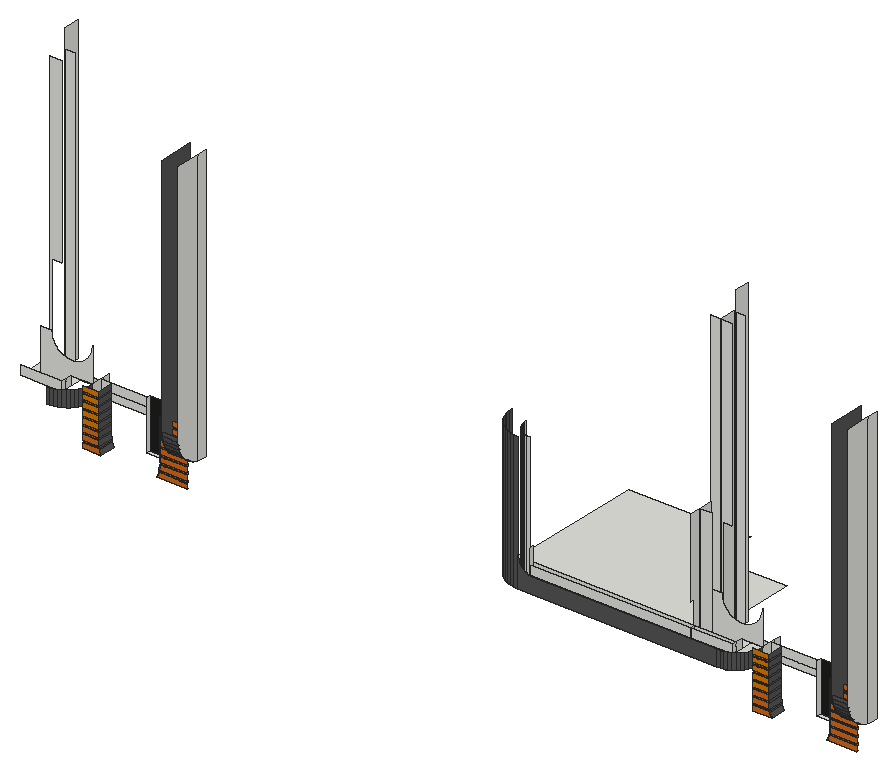
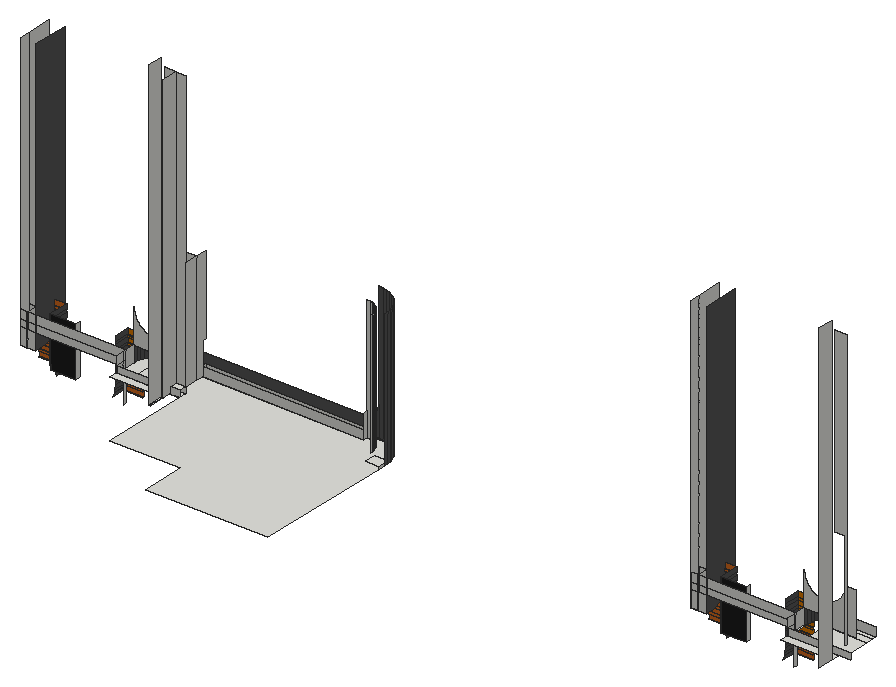
# SketchUp Ruby script. Lengths in inches.
U = 1.inch
M = Sketchup.active_model
def pt(a) = Geom::Point3d.new(a.map { |v| v * U })
def face(e, loops, mat)
  f = e.add_face(loops[0].map { |a| pt(a) })
  loops[1..].each { |l| e.add_face(l.map { |a| pt(a) }).erase! }
  f.material = f.back_material = mat if mat
  f
end
# faces: each face lists its corners as indices into pts; further lists are holes
def faces(e, pts, list, mat = nil) = list.each { |f| face(e, (f[0].is_a?(Array) ? f : [f]).map { |l| l.map { |i| pts[i] } }, mat) }
# xy, xz, yz: faces in a plane at the given z, y or x. An outline is a flat list of corners, or four numbers for a rectangle; further outlines are holes
def ring(l) = l.size == 4 ? [[l[0], l[1]], [l[2], l[1]], [l[2], l[3]], [l[0], l[3]]] : l.each_slice(2).to_a
def flat(e, list, mat, &to3) = list.each { |f| face(e, (f[0].is_a?(Array) ? f : [f]).map { |l| ring(l).map { |u, v| to3.(u, v) } }, mat) }
def xy(e, z, list, mat = nil) = flat(e, list, mat) { |x, y| [x, y, z] }
def xz(e, y, list, mat = nil) = flat(e, list, mat) { |x, z| [x, y, z] }
def yz(e, x, list, mat = nil) = flat(e, list, mat) { |y, z| [x, y, z] }
def lines(e, pts, list) = list.each { |a, b| e.add_line(pt(pts[a]), pt(pts[b])) }
# prism: a flat outline (further loops are holes) pulled along v
def prism(e, loops, v, mat = nil)
  f = face(e, loops, mat); d = Geom::Vector3d.new(v.map { |x| x * U })
  f.pushpull(f.normal.samedirection?(d) ? d.length : -d.length)
end
def box(e, o, s, mat = nil) = prism(e, [[o, [o[0] + s[0], o[1], o[2]], [o[0] + s[0], o[1] + s[1], o[2]], [o[0], o[1] + s[1], o[2]]]], [0, 0, s[2]], mat)
def at(x, y, z, deg = 0) = Geom::Transformation.translation(pt([x, y, z])) * Geom::Transformation.rotation(ORIGIN, Z_AXIS, deg.degrees)
def axes(o, x, y, z) = Geom::Transformation.new([*x, 0, *y, 0, *z, 0, *pt(o).to_a, 1])
def part(name) = M.definitions.add(name)
# library, detail: a bought-in or finely detailed component or shape, given as its bounding box
def library(name, o, s) = part(name).tap { |d| box(d.entities, o, s) }
def detail(e, o, s) = box(e.add_group.entities, o, s)
def put(e, d, t, mat = nil) = e.add_instance(d, t).tap { |i| i.material = mat if mat }
def group(e, t, mat = nil) = e.add_group.tap { |g| g.transformation = t; g.material = mat if mat }.entities
root = M.entities
M.materials.add("[0039_DarkOrange]").color = [219, 120, 0]
M.materials.add("[0041_Chocolate]").color = [210, 105, 30]
M.materials.add("[Color M06]").color = [84, 84, 84]
M.materials.add("[Color M08]").color = [30, 30, 30]
xy(root,90.875,[[1547.71,280.47,1565.89,281.47],[1619.87,280.47,1649.14,281.47],[2198.21,280.47,2216.39,281.47],[2270.37,280.47,2299.64,281.47]],"[0041_Chocolate]")
xy(root,95.83,[[1547.71,280.47,1564.03,281.47],[1621.74,280.47,1649.14,281.47],[2198.21,280.47,2214.53,281.47],[2272.24,280.47,2299.64,281.47]],"[0041_Chocolate]")
xy(root,97.27,[[1597.48,295.65,1621.93,300.34],[2247.98,295.65,2272.43,300.34]])
xy(root,97.9375,[[1547.71,280.47,1563.75,281.47],[1622.02,280.47,1649.14,281.47],[2198.21,280.47,2214.25,281.47],[2272.52,280.47,2299.64,281.47]],"[0041_Chocolate]")
xy(root,102.89,[[1547.71,280.47,1563.1,281.47],[1622.67,280.47,1649.14,281.47],[2198.21,280.47,2213.6,281.47],[2273.17,280.47,2299.64,281.47]],"[0041_Chocolate]")
xy(root,105,[[1547.71,280.47,1563.1,281.47],[1622.67,280.47,1649.14,281.47],[2198.21,280.47,2213.6,281.47],[2273.17,280.47,2299.64,281.47]],"[0041_Chocolate]")
xy(root,109.9375,[[1634.68,299.11,1650.02,302.46],[2285.18,299.11,2300.52,302.46]])
xy(root,109.95,[[1547.71,280.47,1563.1,281.47],[1622.67,280.47,1649.14,281.47],[2198.21,280.47,2213.6,281.47],[2273.17,280.47,2299.64,281.47]],"[0041_Chocolate]")
xy(root,112.0625,[[1547.71,280.47,1563.1,281.47],[2198.21,280.47,2213.6,281.47]],"[0039_DarkOrange]")
xy(root,112.0625,[[1622.67,280.47,1649.14,281.47],[2273.17,280.47,2299.64,281.47]],"[0041_Chocolate]")
xy(root,117.02,[[1547.71,280.47,1563.1,281.47],[2198.21,280.47,2213.6,281.47]],"[0039_DarkOrange]")
xy(root,117.02,[[1622.67,280.47,1649.14,281.47],[2273.17,280.47,2299.64,281.47]],"[0041_Chocolate]")
xy(root,119.125,[[1547.71,280.47,1563.1,281.47],[2198.21,280.47,2213.6,281.47]],"[0039_DarkOrange]")
xy(root,119.125,[[1622.67,280.47,1649.14,281.47],[2273.17,280.47,2299.64,281.47]],"[0041_Chocolate]")
xy(root,124.08,[[1547.71,280.47,1563.1,281.47],[2198.21,280.47,2213.6,281.47]],"[0039_DarkOrange]")
xy(root,124.08,[[1622.67,280.47,1649.14,281.47],[2273.17,280.47,2299.64,281.47]],"[0041_Chocolate]")
xy(root,126.125,[[1980.54,267.75,1976.54,268.01,1972.61,268.79,1970.16,269.625,2182.95,269.625,2179.9,268.59,2176.73,267.96,2173.51,267.75],[1970.16,269.625,1968.8125,270.08,1965.22,271.85,1961.88,274.08,1958.87,276.72,1957.13,278.71,1956.23,279.74,1954,283.07,1952.23,286.66,1950.94,290.46,1950.16,294.39,1949.9,298.39,1949.9,439.98,2068.38,439.98,2068.38,397.86,2137,397.86,2137,305.58,2146.71,305.58,2146.71,312.8125,2198.21,312.8125,2198.21,305.58,2197.71,305.58,2197.71,292.45,2198.21,292.45,2198,289.23,2197.37,286.06,2196.33,283,2194.9,280.1,2193.11,277.41,2190.98,274.98,2188.55,272.85,2185.86,271.06,2182.96,269.63,2182.95,269.625],[1547.21,292.45,1547.71,302.46],[2197.71,292.45,2198.21,302.46],[1547.21,302.46,1547.71,305.58],
  [2197.71,302.46,2198.21,305.58],[2137,305.58,2146.71,312.8125],[1498.09,312.8125,1507.74,321.34],[1507.74,312.8125,1547.71,321.34],[2146.71,312.8125,2147.02,321.34],
  [2147.02,312.8125,2148.59,321.34],[2148.59,312.8125,2158.24,321.34],[2158.24,312.8125,2198.21,321.34],[2146.71,321.34,2147.02,336.27],[2147.02,321.34,2148.59,336.27]])
xy(root,126.1875,[[1547.71,280.47,1563.1,281.47],[2198.21,280.47,2213.6,281.47]],"[0039_DarkOrange]")
xy(root,126.1875,[[1622.67,280.47,1649.14,281.47],[2273.17,280.47,2299.64,281.47]],"[0041_Chocolate]")
xy(root,128.75,[[1949.9,294.33,1962.9,305.58]])
xy(root,131.14,[[1547.71,280.47,1563.1,281.47],[2198.21,280.47,2213.6,281.47]],"[0039_DarkOrange]")
xy(root,131.14,[[1622.67,280.47,1649.14,281.47],[2273.17,280.47,2299.64,281.47]],"[0041_Chocolate]")
xy(root,132.47,[[1486.5,281.47,1527.09,285.84],[1980.54,281.47,2137,285.84],[2137,281.47,2177.59,285.84],[1486.5,285.84,1527.09,292.45],[2137,285.84,2177.59,292.45],
  [1486.5,292.45,1527.09,312.8125],[2137,292.45,2177.59,312.8125]])
xy(root,133.25,[[1547.71,280.47,1563.1,281.47],[2198.21,280.47,2213.6,281.47]],"[0039_DarkOrange]")
xy(root,133.25,[[1622.67,280.47,1649.14,281.47],[2273.17,280.47,2299.64,281.47]],"[0041_Chocolate]")
xy(root,138.2,[[1547.71,280.47,1563.1,281.47],[2198.21,280.47,2213.6,281.47]],"[0039_DarkOrange]")
xy(root,138.2,[[1622.67,280.47,1649.14,281.47],[2273.17,280.47,2299.64,281.47]],"[0041_Chocolate]")
xy(root,140.3125,[[1547.71,280.47,1563.1,281.47],[2198.21,280.47,2213.6,281.47]],"[0039_DarkOrange]")
xy(root,140.3125,[[1622.67,280.47,1649.14,281.47],[2273.17,280.47,2299.64,281.47]],"[0041_Chocolate]")
xz(root,267.75,[[1980.54,126.125,2173.51,126.125,2173.51,141.26,1993.98,141.26,1992.2,141.46,1990.46,141.89,1988.79,142.53,1987.21,143.38,1985.75,144.42,1984.43,145.64,1983.28,147.01,1982.32,148.52,1981.55,150.14,1980.99,151.84,1980.65,153.6,1980.54,155.39]],"[Color M06]")
xz(root,280.47,[[1547.71,112.0625,1563.1,117.02],[2198.21,112.0625,2213.6,117.02],[1547.71,119.125,1563.1,124.08],[2198.21,119.125,2213.6,124.08],[1547.71,126.1875,1563.1,131.14],
  [2198.21,126.1875,2213.6,131.14],[1547.71,133.25,1563.1,138.2],[2198.21,133.25,2213.6,138.2],[1547.71,140.3125,1563.1,145.27],[2198.21,140.3125,2213.6,145.27]],"[0039_DarkOrange]")
xz(root,280.47,[[1547.71,90.875,1565.89,90.875,1564.11,95.18,1564.03,95.83,1547.71,95.83],[1619.87,90.875,1649.14,90.875,1649.14,95.83,1621.74,95.83,1621.66,95.18],[2198.21,90.875,2216.39,90.875,2214.61,95.18,2214.53,95.83,2198.21,95.83],[2270.37,90.875,2299.64,90.875,2299.64,95.83,2272.24,95.83,2272.16,95.18],[1547.71,97.9375,1563.75,97.9375,1563.1,102.89,1547.71,102.89],
  [1622.02,97.9375,1649.14,97.9375,1649.14,102.89,1622.67,102.89],[2198.21,97.9375,2214.25,97.9375,2213.6,102.89,2198.21,102.89],[2272.52,97.9375,2299.64,97.9375,2299.64,102.89,2273.17,102.89],[1547.71,105,1563.1,109.95],[1622.67,105,1649.14,109.95],
  [2198.21,105,2213.6,109.95],[2273.17,105,2299.64,109.95],[1622.67,112.0625,1649.14,117.02],[2273.17,112.0625,2299.64,117.02],[1622.67,119.125,1649.14,124.08],
  [2273.17,119.125,2299.64,124.08],[1622.67,126.1875,1649.14,131.14],[2273.17,126.1875,2299.64,131.14],[1622.67,133.25,1649.14,138.2],[2273.17,133.25,2299.64,138.2],
  [1622.67,140.3125,1649.14,145.27],[2273.17,140.3125,2299.64,145.27]],"[0041_Chocolate]")
xz(root,281.47,[[1486.5,132.47,1527.09,141.26],[1980.54,132.47,2137,141.26],[2137,132.47,2177.59,141.26]])
xz(root,281.47,[[1547.71,117.02,1563.1,119.125],[2198.21,117.02,2213.6,119.125],[1547.71,124.08,1563.1,126.1875],[2198.21,124.08,2213.6,126.1875],[1547.71,131.14,1563.1,133.25],
  [2198.21,131.14,2213.6,133.25],[1547.71,138.2,1563.1,140.3125],[2198.21,138.2,2213.6,140.3125]],"[0039_DarkOrange]")
xz(root,281.47,[[1547.71,95.83,1564.03,95.83,1563.75,97.9375,1547.71,97.9375],[1621.74,95.83,1649.14,95.83,1649.14,97.9375,1622.02,97.9375],[2198.21,95.83,2214.53,95.83,2214.25,97.9375,2198.21,97.9375],[2272.24,95.83,2299.64,95.83,2299.64,97.9375,2272.52,97.9375],[1547.71,102.89,1563.1,105],
  [1622.67,102.89,1649.14,105],[2198.21,102.89,2213.6,105],[2273.17,102.89,2299.64,105],[1547.71,109.95,1563.1,112.0625],[1622.67,109.95,1649.14,112.0625],
  [2198.21,109.95,2213.6,112.0625],[2273.17,109.95,2299.64,112.0625],[1622.67,117.02,1649.14,119.125],[2273.17,117.02,2299.64,119.125],[1622.67,124.08,1649.14,126.1875],
  [2273.17,124.08,2299.64,126.1875],[1622.67,131.14,1649.14,133.25],[2273.17,131.14,2299.64,133.25],[1622.67,138.2,1649.14,140.3125],[2273.17,138.2,2299.64,140.3125]],"[0041_Chocolate]")
xz(root,285.84,[[1980.54,132.47,2177.59,141.26]])
xz(root,292.45,[[1642.35,126.125,1643.23,141.26],[1643.23,126.125,1649.14,141.26],[2292.85,126.125,2293.73,141.26],[2293.73,126.125,2299.64,141.26],[1498.09,132.47,1527.09,132.47,1527.09,141.26,1547.71,141.26,1547.71,174.51,1547.68,173.46,1547.6,172.42,1547.46,171.38,1547.27,170.36,1547.03,169.34,1546.73,168.33,1546.38,167.35,1545.98,166.38,1545.53,165.4375,1545.03,164.52,1544.49,163.625,1543.89,162.76,1543.26,161.93,1542.58,161.14,1541.86,160.38,1541.1,159.66,1540.3,158.98,1539.47,158.34,1538.61,157.75,1537.72,157.2,1536.8,156.7,1535.86,156.25,1534.89,155.85,1533.9,155.5,1532.9,155.21,1531.88,154.96,1530.85,154.77,1529.82,154.64,1528.77,154.55,1527.73,154.53,1526.68,154.55,1525.64,154.64,1524.6,154.77,1523.57,154.96,1522.55,155.21,1521.55,155.5,1520.57,155.85,1519.6,156.25,1518.65,156.7,1517.73,157.2,1516.84,157.75,1515.98,158.34,1515.15,158.98,1514.35,159.66,1513.6,160.38,1512.875,161.14,1512.2,161.93,1511.56,162.76,1510.97,163.625,1510.42,164.52,1509.92,165.4375,1509.47,166.38,1509.07,167.35,1508.72,168.33,1508.42,169.34,1508.18,170.36,1507.99,171.38,1507.85,172.42,1507.77,173.46,1507.74,174.51,1498.09,174.51],
  [2137,132.47,2148.59,240.16],[2148.59,132.47,2177.59,132.47,2177.59,141.26,2198.21,141.26,2198.21,174.51,2198.18,173.46,2198.1,172.42,2197.96,171.38,2197.77,170.36,2197.53,169.34,2197.23,168.33,2196.88,167.35,2196.48,166.38,2196.03,165.4375,2195.53,164.52,2194.99,163.625,2194.39,162.76,2193.76,161.93,2193.08,161.14,2192.36,160.38,2191.6,159.66,2190.8,158.98,2189.97,158.34,2189.11,157.75,2188.22,157.2,2187.3,156.7,2186.36,156.25,2185.39,155.85,2184.4,155.5,2183.4,155.21,2182.38,154.96,2181.35,154.77,2180.32,154.64,2179.27,154.55,2178.23,154.53,2177.18,154.55,2176.14,154.64,2175.1,154.77,2174.07,154.96,2173.05,155.21,2172.05,155.5,2171.07,155.85,2170.1,156.25,2169.15,156.7,2168.23,157.2,2167.34,157.75,2166.48,158.34,2165.65,158.98,2164.85,159.66,2164.1,160.38,2163.375,161.14,2162.7,161.93,2162.06,162.76,2161.47,163.625,2160.92,164.52,2160.42,165.4375,2159.97,166.38,2159.57,167.35,2159.22,168.33,2158.92,169.34,2158.68,170.36,2158.49,171.38,2158.35,172.42,2158.27,173.46,2158.24,174.51,2148.59,174.51]])
xz(root,295.65,[[1621.93,97.27,1622.67,97.27,1622.67,102.89,1622.02,97.9375],[2272.43,97.27,2273.17,97.27,2273.17,102.89,2272.52,97.9375]])
xz(root,300.34,[[1597.48,97.27,1621.93,97.27,1622.02,97.9375,1622.67,102.89,1622.67,145.27,1597.48,145.27],[2247.98,97.27,2272.43,97.27,2272.52,97.9375,2273.17,102.89,2273.17,145.27,2247.98,145.27]],"[Color M08]")
xz(root,302.46,[[1547.21,95.62,1547.71,126.125],[2197.71,95.62,2198.21,126.125],[1634.68,109.9375,1642.35,126.125],[1642.35,109.9375,1643.23,126.125],[1643.23,109.9375,1650.02,126.125],
  [2285.18,109.9375,2292.85,126.125],[2292.85,109.9375,2293.73,126.125],[2293.73,109.9375,2300.52,126.125],[1547.71,126.125,1634.68,132.47],[1634.68,126.125,1642.35,132.47],
  [1642.35,126.125,1643.23,132.47],[1643.23,126.125,1650.02,132.47],[2198.21,126.125,2285.18,132.47],[2285.18,126.125,2292.85,132.47],[2292.85,126.125,2293.73,132.47],
  [2293.73,126.125,2300.52,132.47],[1547.71,132.47,1634.68,141.26],[1634.68,132.47,1642.35,141.26],[1642.35,132.47,1643.23,141.26],[1643.23,132.47,1650.02,141.26],
  [2198.21,132.47,2285.18,141.26],[2285.18,132.47,2292.85,141.26],[2292.85,132.47,2293.73,141.26],[2293.73,132.47,2300.52,141.26]])
xz(root,305.58,[[1496.21,126.125,1498.09,126.125,1498.09,226.8,1507.74,226.8,1507.74,402.64,1496.21,402.64],[2137,126.125,2146.71,402.64],[2146.71,126.125,2148.59,126.125,2148.59,226.8,2158.24,226.8,2158.24,402.64,2146.71,402.64]])
xz(root,312.8125,[[1486.5,126.125,1547.71,132.47],[2137,126.125,2198.21,132.47]])
xz(root,321.34,[[1498.09,126.125,1507.74,402.64],[2146.71,126.125,2148.59,402.64],[2148.59,126.125,2158.24,402.64]])
yz(root,1498.09,[[321.34,126.125,336.27,421.25]])
yz(root,1527.09,[[281.47,132.47,285.84,141.26],[285.84,132.47,292.45,141.26]])
yz(root,1547.21,[[302.46,95.62,305.58,126.125]])
yz(root,1547.71,[[292.45,126.125,302.46,141.26],[302.46,126.125,305.58,132.47],[305.58,126.125,312.8125,132.47],[302.46,132.47,305.58,141.26],[305.58,132.47,312.8125,141.26]])
yz(root,1563.1,[[281.47,102.89,295.65,105],[280.47,105,295.65,109.95],[281.47,109.95,295.65,112.0625],[280.47,112.0625,295.65,117.02],[281.47,117.02,295.65,119.125],
  [280.47,119.125,295.65,124.08],[281.47,124.08,295.65,126.1875],[280.47,126.1875,295.65,131.14],[281.47,131.14,295.65,133.25],[280.47,133.25,295.65,138.2],
  [281.47,138.2,295.65,140.3125],[280.47,140.3125,295.65,145.27]],"[Color M06]")
yz(root,1597.48,[[295.65,97.27,300.34,145.27]])
yz(root,1622.67,[[281.47,102.89,300.34,105],[280.47,105,300.34,109.95],[281.47,109.95,300.34,112.0625],[280.47,112.0625,300.34,117.02],[281.47,117.02,300.34,119.125],
  [280.47,119.125,300.34,124.08],[281.47,124.08,300.34,126.1875],[280.47,126.1875,300.34,131.14],[281.47,131.14,300.34,133.25],[280.47,133.25,300.34,138.2],
  [281.47,138.2,300.34,140.3125],[280.47,140.3125,300.34,145.27]],"[Color M06]")
yz(root,1634.68,[[299.11,109.9375,295.02,110.21,290.99,111.01,287.11,112.32,283.43,114.14,280.02,116.42,276.93,119.12,274.23,122.21,271.95,125.62,270.14,129.3,268.82,133.18,268.02,137.2,267.75,141.3,267.75,376.875,302.46,376.875,302.46,109.9375]],"[Color M06]")
yz(root,1642.35,[[292.45,126.125,302.46,141.26]])
yz(root,1650.02,[[299.11,109.9375,302.46,109.9375,302.46,376.875,292.45,376.875,292.45,110.72,295.02,110.21],[299.11,109.9375,302.46,109.9375,302.46,376.875,292.45,376.875,292.45,110.72,295.02,110.21],[292.45,110.72,292.45,376.875,267.75,376.875,267.75,141.3,268.02,137.2,268.82,133.18,270.14,129.3,271.95,125.62,274.23,122.21,276.93,119.12,280.02,116.42,283.43,114.14,287.11,112.32,290.99,111.01]])
yz(root,1949.9,[[298.39,126.125,305.58,128.75]])
yz(root,1980.54,[[281.47,132.47,285.84,155.39]])
yz(root,2137,[[281.47,132.47,281.47,141.26,285.84,141.26,285.84,163.7,281.47,163.7,281.47,240.16,292.45,240.16,292.45,132.47],[292.45,132.47,305.58,240.16]])
yz(root,2146.71,[[305.58,126.125,321.34,402.64]])
yz(root,2148.59,[[321.34,126.125,336.27,421.25]])
yz(root,2177.59,[[281.47,132.47,285.84,141.26],[285.84,132.47,292.45,141.26]])
yz(root,2197.71,[[302.46,95.62,305.58,126.125]])
yz(root,2198.21,[[292.45,126.125,302.46,141.26],[302.46,126.125,305.58,132.47],[305.58,126.125,312.8125,132.47],[302.46,132.47,305.58,141.26],[305.58,132.47,312.8125,141.26]])
yz(root,2213.6,[[281.47,102.89,295.65,105],[280.47,105,295.65,109.95],[281.47,109.95,295.65,112.0625],[280.47,112.0625,295.65,117.02],[281.47,117.02,295.65,119.125],
  [280.47,119.125,295.65,124.08],[281.47,124.08,295.65,126.1875],[280.47,126.1875,295.65,131.14],[281.47,131.14,295.65,133.25],[280.47,133.25,295.65,138.2],
  [281.47,138.2,295.65,140.3125],[280.47,140.3125,295.65,145.27]],"[Color M06]")
yz(root,2247.98,[[295.65,97.27,300.34,145.27]])
yz(root,2273.17,[[281.47,102.89,300.34,105],[280.47,105,300.34,109.95],[281.47,109.95,300.34,112.0625],[280.47,112.0625,300.34,117.02],[281.47,117.02,300.34,119.125],
  [280.47,119.125,300.34,124.08],[281.47,124.08,300.34,126.1875],[280.47,126.1875,300.34,131.14],[281.47,131.14,300.34,133.25],[280.47,133.25,300.34,138.2],
  [281.47,138.2,300.34,140.3125],[280.47,140.3125,300.34,145.27]],"[Color M06]")
yz(root,2285.18,[[299.11,109.9375,295.02,110.21,290.99,111.01,287.11,112.32,283.43,114.14,280.02,116.42,276.93,119.12,274.23,122.21,271.95,125.62,270.14,129.3,268.82,133.18,268.02,137.2,267.75,141.3,267.75,376.875,302.46,376.875,302.46,109.9375]],"[Color M06]")
yz(root,2292.85,[[292.45,126.125,302.46,141.26]])
yz(root,2300.52,[[299.11,109.9375,302.46,109.9375,302.46,376.875,292.45,376.875,292.45,110.72,295.02,110.21],[292.45,110.72,292.45,376.875,267.75,376.875,267.75,141.3,268.02,137.2,268.82,133.18,270.14,129.3,271.95,125.62,274.23,122.21,276.93,119.12,280.02,116.42,283.43,114.14,287.11,112.32,290.99,111.01]])
p = [[1564.11,295.65,95.18],[1564.11,280.47,95.18],[1565.89,280.47,90.875],[1565.89,281.47,90.875],[1565.89,295.65,90.875],[1619.87,295.65,90.875],
  [1619.87,281.47,90.875],[1619.87,280.47,90.875],[1621.66,280.47,95.18],[1621.66,295.65,95.18],[2214.61,295.65,95.18],[2214.61,280.47,95.18],
  [2216.39,280.47,90.875],[2216.39,281.47,90.875],[2216.39,295.65,90.875],[2270.37,295.65,90.875],[2270.37,281.47,90.875],[2270.37,280.47,90.875],
  [2272.16,280.47,95.18],[2272.16,295.65,95.18],[1564.03,295.65,95.83],[1564.03,281.47,95.83],[1564.03,280.47,95.83],[1621.74,280.47,95.83],
  [1621.74,281.47,95.83],[1621.74,295.65,95.83],[2214.53,295.65,95.83],[2214.53,281.47,95.83],[2214.53,280.47,95.83],[2272.24,280.47,95.83],
  [2272.24,281.47,95.83],[2272.24,295.65,95.83],[1563.75,281.47,97.9375],[1563.75,295.65,97.9375],[1622.02,281.47,97.9375],[1622.02,295.65,97.9375],
  [1621.93,295.65,97.27],[2214.25,281.47,97.9375],[2214.25,295.65,97.9375],[2272.52,281.47,97.9375],[2272.52,295.65,97.9375],[2272.43,295.65,97.27],
  [1622.02,300.34,97.9375],[1621.93,300.34,97.27],[2272.52,300.34,97.9375],[2272.43,300.34,97.27],[1563.1,295.65,102.89],[1563.1,281.47,102.89],
  [1563.1,280.47,102.89],[1563.75,280.47,97.9375],[1622.02,280.47,97.9375],[1622.67,280.47,102.89],[1622.67,281.47,102.89],[1622.67,295.65,102.89],
  [2213.6,295.65,102.89],[2213.6,281.47,102.89],[2213.6,280.47,102.89],[2214.25,280.47,97.9375],[2272.52,280.47,97.9375],[2273.17,280.47,102.89],
  [2273.17,281.47,102.89],[2273.17,295.65,102.89],[1622.67,300.34,102.89],[2273.17,300.34,102.89],[1650.02,299.11,109.9375],[1650.02,295.02,110.21],
  [1634.68,295.02,110.21],[1634.68,299.11,109.9375],[2300.52,299.11,109.9375],[2300.52,295.02,110.21],[2285.18,295.02,110.21],[2285.18,299.11,109.9375],
  [1650.02,292.45,110.72],[1650.02,290.99,111.01],[1634.68,290.99,111.01],[2300.52,292.45,110.72],[2300.52,290.99,111.01],[2285.18,290.99,111.01],
  [1650.02,287.11,112.32],[1634.68,287.11,112.32],[2300.52,287.11,112.32],[2285.18,287.11,112.32],[1650.02,283.43,114.14],[1634.68,283.43,114.14],
  [2300.52,283.43,114.14],[2285.18,283.43,114.14],[1650.02,280.02,116.42],[1634.68,280.02,116.42],[2300.52,280.02,116.42],[2285.18,280.02,116.42],
  [1650.02,276.93,119.12],[1634.68,276.93,119.12],[2300.52,276.93,119.12],[2285.18,276.93,119.12],[1650.02,274.23,122.21],[1634.68,274.23,122.21],
  [2300.52,274.23,122.21],[2285.18,274.23,122.21],[1650.02,271.95,125.62],[1634.68,271.95,125.62],[2300.52,271.95,125.62],[2285.18,271.95,125.62],
  [1650.02,270.14,129.3],[1634.68,270.14,129.3],[2300.52,270.14,129.3],[2285.18,270.14,129.3],[1526.23,267.96,141.26],[1523.01,267.75,141.26],
  [1523.01,267.75,126.125],[1526.23,267.96,126.125],[1980.54,267.75,258.13],[1976.54,268.01,258.13],[1976.54,268.01,126.125],[1980.54,267.75,126.125],
  [1980.54,267.75,155.39],[1980.54,267.75,164.97],[1980.54,267.75,240.16],[2176.73,267.96,141.26],[2173.51,267.75,141.26],[2173.51,267.75,126.125],
  [2176.73,267.96,126.125],[1529.4,268.59,141.26],[1529.4,268.59,126.125],[1972.61,268.79,258.13],[1972.61,268.79,126.125],[2179.9,268.59,141.26],
  [2179.9,268.59,126.125],[1532.46,269.63,141.26],[1532.45,269.625,126.125],[1532.46,269.63,126.125],[2182.96,269.63,141.26],[2182.95,269.625,126.125],
  [2182.96,269.63,126.125],[1968.8125,270.08,258.13],[1968.8125,270.08,126.125],[1970.16,269.625,126.125],[1535.36,271.06,141.26],[1535.36,271.06,126.125],
  [2185.86,271.06,141.26],[2185.86,271.06,126.125],[1965.22,271.85,258.13],[1965.22,271.85,126.125],[1538.05,272.85,141.26],[1538.05,272.85,126.125],
  [2188.55,272.85,141.26],[2188.55,272.85,126.125],[1961.88,274.08,258.13],[1961.88,274.08,126.125],[1540.48,274.98,141.26],[1540.48,274.98,126.125],
  [2190.98,274.98,141.26],[2190.98,274.98,126.125],[1958.87,276.72,258.13],[1958.87,276.72,126.125],[1542.61,277.41,141.26],[1542.61,277.41,126.125],
  [2193.11,277.41,141.26],[2193.11,277.41,126.125],[1956.23,279.74,258.13],[1956.23,279.74,126.125],[1957.13,278.71,126.125],[1544.4,280.1,141.26],
  [1544.4,280.1,126.125],[2194.9,280.1,141.26],[2194.9,280.1,126.125],[1954,283.07,258.13],[1954,283.07,126.125],[1545.07,281.47,141.26],
  [1545.83,283,126.125],[1545.83,283,141.26],[2195.57,281.47,141.26],[2196.33,283,126.125],[2196.33,283,141.26],[1546.87,286.06,141.26],
  [1546.87,286.06,126.125],[2197.37,286.06,141.26],[2197.37,286.06,126.125],[1952.23,286.66,258.13],[1952.23,286.66,126.125],[1547.5,289.23,141.26],
  [1547.5,289.23,126.125],[2198,289.23,141.26],[2198,289.23,126.125],[1950.94,290.46,258.13],[1950.94,290.46,126.125],[1547.71,292.45,141.26],
  [1547.71,292.45,126.125],[2198.21,292.45,141.26],[2198.21,292.45,126.125],[1950.16,294.39,258.13],[1950.16,294.39,126.125],[1949.9,298.39,240.16],
  [1949.9,298.39,132.47],[1949.9,298.39,128.75],[1949.9,298.39,126.125],[1949.9,298.39,258.13],[1650.02,268.82,133.18],[1634.68,268.82,133.18],
  [2300.52,268.82,133.18],[2285.18,268.82,133.18],[1978.33,281.61,252.47],[1980.54,281.47,252.47],[1980.54,281.47,240.16],[1980.54,281.47,164.97],
  [1980.54,281.47,163.7],[1980.54,281.47,155.39],[1980.54,281.47,141.26],[1980.54,281.47,132.47],[1978.33,281.61,132.47],[1976.16,282.04,252.47],
  [1976.16,282.04,132.47],[1974.06,282.75,252.47],[1974.06,282.75,132.47],[1972.07,283.73,252.47],[1972.07,283.73,132.47],[1970.23,284.96,252.47],
  [1970.23,284.96,132.47],[1968.57,286.42,252.47],[1968.57,286.42,132.47],[1967.11,288.09,252.47],[1967.11,288.09,132.47],[1965.88,289.93,252.47],
  [1965.88,289.93,132.47],[1964.9,291.91,252.47],[1964.9,291.91,132.47],[1964.1875,294.01,252.47],[1964.1875,294.01,132.47],[1963.76,296.18,252.47],
  [1963.76,296.18,132.47],[1963.61,298.39,252.47],[1963.61,298.39,132.47],[1963.61,298.39,240.16],[1650.02,268.02,137.2],[1634.68,268.02,137.2],
  [2300.52,268.02,137.2],[2285.18,268.02,137.2],[1650.02,267.75,141.3],[1634.68,267.75,141.3],[2300.52,267.75,141.3],[2285.18,267.75,141.3]]
faces(root,p,[[0,1,2,3,4],[5,6,7,8,9],[10,11,12,13,14],[15,16,17,18,19],[20,21,22,1,0],[9,8,23,24,25],[26,27,28,11,10],[19,18,29,30,31],
  [32,21,20,33],[24,34,35,36,25],[37,27,26,38],[30,39,40,41,31],[46,47,48,49,32,33],[35,34,50,51,52,53],[54,55,56,57,37,38],[40,39,58,59,60,61],
  [35,53,62,42],[40,61,63,44],[64,65,66,67],[68,69,70,71],[72,73,74,66,65],[75,76,77,70,69],[73,78,79,74],[76,80,81,77],
  [78,82,83,79],[80,84,85,81],[82,86,87,83],[84,88,89,85],[86,90,91,87],[88,92,93,89],[90,94,95,91],[92,96,97,93],
  [94,98,99,95],[96,100,101,97],[98,102,103,99],[100,104,105,101],[106,107,108,109],[110,111,112,113,114,115,116],[117,118,119,120],[121,106,109,122],
  [111,123,124,112],[125,117,120,126],[127,121,122,128,129],[130,125,126,131,132],[133,134,135,124,123],[136,127,129,137],[138,130,132,139],[140,141,134,133],
  [142,136,137,143],[144,138,139,145],[146,147,141,140],[148,142,143,149],[150,144,145,151],[152,153,147,146],[154,148,149,155],[156,150,151,157],
  [158,159,160,153,152],[161,154,155,162],[163,156,157,164],[165,166,159,158],[167,161,162,168,169],[170,163,164,171,172],[173,169,168,174],[175,172,171,176],
  [177,178,166,165],[179,173,174,180],[181,175,176,182],[183,184,178,177],[185,179,180,186],[187,181,182,188],[189,190,184,183],[191,192,193,194,190,189,195],
  [102,196,197,103],[104,198,199,105],[196,232,233,197],[198,234,235,199],[232,236,237,233],[234,238,239,235]],"[Color M06]")
faces(root,p,[[36,35,42,43],[41,40,44,45],[200,201,202,203,204,205,206,207,208],[209,200,208,210],[211,209,210,212],[213,211,212,214],[215,213,214,216],[217,215,216,218],
  [219,217,218,220],[221,219,220,222],[223,221,222,224],[225,223,224,226],[227,225,226,228],[229,227,228,230,231]])
